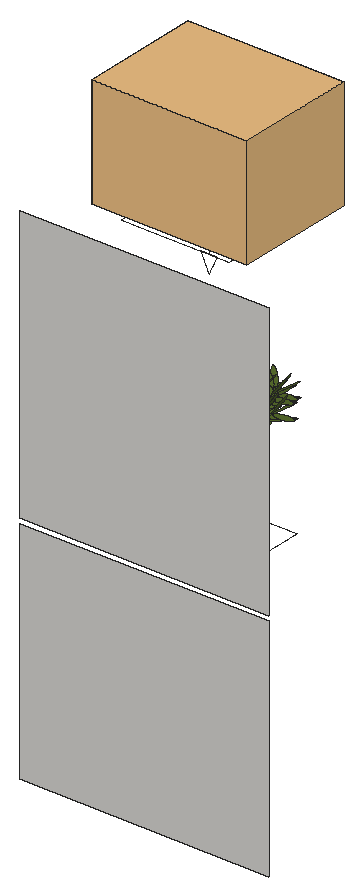
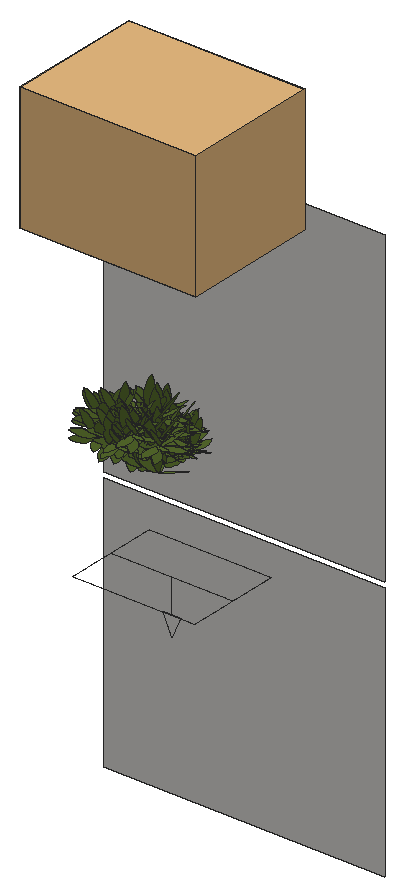
# SketchUp Ruby script. Lengths in inches.
U = 1.inch
M = Sketchup.active_model
def pt(a) = Geom::Point3d.new(a.map { |v| v * U })
def face(e, loops, mat)
  f = e.add_face(loops[0].map { |a| pt(a) })
  loops[1..].each { |l| e.add_face(l.map { |a| pt(a) }).erase! }
  f.material = f.back_material = mat if mat
  f
end
# faces: each face lists its corners as indices into pts; further lists are holes
def faces(e, pts, list, mat = nil) = list.each { |f| face(e, (f[0].is_a?(Array) ? f : [f]).map { |l| l.map { |i| pts[i] } }, mat) }
# xy, xz, yz: faces in a plane at the given z, y or x. An outline is a flat list of corners, or four numbers for a rectangle; further outlines are holes
def ring(l) = l.size == 4 ? [[l[0], l[1]], [l[2], l[1]], [l[2], l[3]], [l[0], l[3]]] : l.each_slice(2).to_a
def flat(e, list, mat, &to3) = list.each { |f| face(e, (f[0].is_a?(Array) ? f : [f]).map { |l| ring(l).map { |u, v| to3.(u, v) } }, mat) }
def xy(e, z, list, mat = nil) = flat(e, list, mat) { |x, y| [x, y, z] }
def xz(e, y, list, mat = nil) = flat(e, list, mat) { |x, z| [x, y, z] }
def yz(e, x, list, mat = nil) = flat(e, list, mat) { |y, z| [x, y, z] }
def lines(e, pts, list) = list.each { |a, b| e.add_line(pt(pts[a]), pt(pts[b])) }
# prism: a flat outline (further loops are holes) pulled along v
def prism(e, loops, v, mat = nil)
  f = face(e, loops, mat); d = Geom::Vector3d.new(v.map { |x| x * U })
  f.pushpull(f.normal.samedirection?(d) ? d.length : -d.length)
end
def box(e, o, s, mat = nil) = prism(e, [[o, [o[0] + s[0], o[1], o[2]], [o[0] + s[0], o[1] + s[1], o[2]], [o[0], o[1] + s[1], o[2]]]], [0, 0, s[2]], mat)
def at(x, y, z, deg = 0) = Geom::Transformation.translation(pt([x, y, z])) * Geom::Transformation.rotation(ORIGIN, Z_AXIS, deg.degrees)
def axes(o, x, y, z) = Geom::Transformation.new([*x, 0, *y, 0, *z, 0, *pt(o).to_a, 1])
def part(name) = M.definitions.add(name)
# library, detail: a bought-in or finely detailed component or shape, given as its bounding box
def library(name, o, s) = part(name).tap { |d| box(d.entities, o, s) }
def detail(e, o, s) = box(e.add_group.entities, o, s)
def put(e, d, t, mat = nil) = e.add_instance(d, t).tap { |i| i.material = mat if mat }
def group(e, t, mat = nil) = e.add_group.tap { |g| g.transformation = t; g.material = mat if mat }.entities
root = M.entities
M.materials.add("[0008_LavenderBlush]").color = [212, 210, 207]
M.materials.add("[Asphalt_New]").color = [85, 106, 44]
M.materials.add("white").color = [255, 255, 255]
c1 = library("Hanging planter",[0,-5.51,0],[18.9,24.41,17.52])
c2 = part("Component\#59")
xy(c2.entities,0,[[5.79,0,4.75,0.06,3.73,0.22,2.73,0.5,1.77,0.88,0.86,1.37,0,1.95,0.83,2.59,1.74,3.13,2.7,3.56,3.7,3.87,4.74,4.05,5.79,4.12,6.84,4.05,7.87,3.87,8.88,3.56,9.84,3.13,10.74,2.59,11.57,1.95,10.72,1.37,9.8,0.88,8.84,0.5,7.84,0.22,6.82,0.06]],"[Asphalt_New]")
c3 = part("Leaf cluster")
put(c3.entities,c2,axes([10.37,9.23,1.73],[-0.67725,-0.67301,0.29729],[0.61625,-0.73963,-0.27052],[0.40195,0,0.91566]),"[Asphalt_New]")
put(c3.entities,c2,at(0,5.84,1.2),"[Asphalt_New]")
put(c3.entities,c2,axes([11.625,9.72,1.52],[-0.61694,-0.11161,0.77906],[-0.02647,-0.98639,-0.16227],[0.78657,-0.12073,0.60559]),"[Asphalt_New]")
put(c3.entities,c2,axes([13.35,8.05,1.98],[-0.1211,0.99122,-0.05316],[-0.90762,-0.13226,-0.39842],[-0.40195,0,0.91566]),"[Asphalt_New]")
c4 = part("Group141\#1")
p = [[0,0,0],[0,0,-2.45],[-0.68,0,-2.45],[4.45,-3.49,0],[-4.45,-3.49,0],[4.45,3.49,0],
  [4.45,0,0],[-4.45,3.49,0],[0.68,0,-2.45],[-4.45,0,0],[0,0,-3.97]]
lines(c4.entities,p,[[0,1],[1,2],[3,4],[5,6],[7,5],[1,8],[9,0],[0,6],[8,10],[4,9],[6,3],[2,10],
  [9,7]])
c5 = part("Rectangle Light")
put(c5.entities,c4,at(0,0,0))
c6 = part("Groupe\#6")
put(c6.entities,c3,axes([6.2,8.72,2.56],[0.20072,0.20931,0],[-0.20931,0.20072,0],[0,0,0.3393]))
put(c6.entities,c3,axes([3.21,14.77,2.82],[0.12393,-0.26218,0],[0.26218,0.12393,0],[0,0,0.3393]))
put(c6.entities,c2,axes([6.98,12.58,2.74],[0.18147,-0.01125,0.26433],[0.07569,0.27597,-0.05506],[-0.21317,0.08841,0.20548]),"[Asphalt_New]")
put(c6.entities,c3,axes([9.62,7.71,2.12],[0.13301,0.2577,0],[-0.2577,0.13301,0],[0,0,0.3393]))
put(c6.entities,c3,axes([5.04,12.65,2.375],[0.19329,-0.21619,0],[0.21619,0.19329,0],[0,0,0.3393]))
put(c6.entities,c3,axes([8.55,8.27,2.12],[0.13301,0.2577,0],[-0.2577,0.13301,0],[0,0,0.3393]))
put(c6.entities,c3,axes([3.97,13.21,2.375],[0.19329,-0.21619,0],[0.21619,0.19329,0],[0,0,0.3393]))
put(c6.entities,c3,axes([13.2,6.93,2.95],[-0.24238,0.15922,0],[-0.15922,-0.24238,0],[0,0,0.3393]))
put(c6.entities,c3,axes([7.8,2.89,3.21],[0.23521,0.16964,0],[-0.16964,0.23521,0],[0,0,0.3393]))
put(c6.entities,c2,axes([9.26,7,3.13],[-0.02201,0.18048,0.26433],[-0.28514,0.02413,-0.05506],[-0.04808,-0.22571,0.20548]),"[Asphalt_New]")
put(c6.entities,c3,axes([10.92,8.49,3.88],[-0.24238,0.15922,0],[-0.15922,-0.24238,0],[0,0,0.3393]))
put(c6.entities,c3,axes([5.52,4.45,4.14],[0.23521,0.16964,0],[-0.16964,0.23521,0],[0,0,0.3393]))
put(c6.entities,c2,axes([6.97,8.56,4.0625],[-0.02201,0.18048,0.26433],[-0.28514,0.02413,-0.05506],[-0.04808,-0.22571,0.20548]),"[Asphalt_New]")
put(c6.entities,c3,axes([9.9,10.06,2.52],[-0.24238,0.15922,0],[-0.15922,-0.24238,0],[0,0,0.3393]))
put(c6.entities,c3,axes([4.51,6.02,2.78],[0.23521,0.16964,0],[-0.16964,0.23521,0],[0,0,0.3393]))
put(c6.entities,c2,axes([5.96,10.125,2.71],[-0.02201,0.18048,0.26433],[-0.28514,0.02413,-0.05506],[-0.04808,-0.22571,0.20548]),"[Asphalt_New]")
put(c6.entities,c3,axes([13.6,14.86,2.41],[-0.24779,-0.15066,0],[0.15066,-0.24779,0],[0,0,0.3393]))
put(c6.entities,c3,axes([8.65,12.2,2.15],[0.22914,-0.17774,0],[0.17774,0.22914,0],[0,0,0.3393]))
put(c6.entities,c3,axes([14.35,15.81,2.41],[-0.24779,-0.15066,0],[0.15066,-0.24779,0],[0,0,0.3393]))
put(c6.entities,c3,axes([7.9,11.25,2.15],[0.22914,-0.17774,0],[0.17774,0.22914,0],[0,0,0.3393]))
put(c6.entities,c3,axes([-0.46,12.1,3.24],[0.12393,-0.26218,0],[0.26218,0.12393,0],[0,0,0.3393]))
put(c6.entities,c2,axes([3.31,9.91,3.17],[0.18147,-0.01125,0.26433],[0.07569,0.27597,-0.05506],[-0.21317,0.08841,0.20548]),"[Asphalt_New]")
put(c6.entities,c3,axes([4.47,8.01,3.91],[0.20072,0.20931,0],[-0.20931,0.20072,0],[0,0,0.3393]))
put(c6.entities,c3,axes([1.49,14.06,4.17],[0.12393,-0.26218,0],[0.26218,0.12393,0],[0,0,0.3393]))
put(c6.entities,c2,axes([5.26,11.88,4.1],[0.18147,-0.01125,0.26433],[0.07569,0.27597,-0.05506],[-0.21317,0.08841,0.20548]),"[Asphalt_New]")
put(c6.entities,c3,axes([6.85,4.1,2.54],[0.13301,0.2577,0],[-0.2577,0.13301,0],[0,0,0.3393]))
put(c6.entities,c3,axes([2.27,9.05,2.8],[0.19329,-0.21619,0],[0.21619,0.19329,0],[0,0,0.3393]))
put(c6.entities,c2,axes([6.51,8.03,2.73],[0.17719,0.04076,0.26433],[-0.00581,0.2861,-0.05506],[-0.2295,0.02423,0.20548]),"[Asphalt_New]")
put(c6.entities,c3,axes([4.86,14.63,2.58],[0.22914,-0.17774,0],[0.17774,0.22914,0],[0,0,0.3393]))
put(c6.entities,c3,axes([10.5625,18.23,2.83],[-0.24779,-0.15066,0],[0.15066,-0.24779,0],[0,0,0.3393]))
put(c6.entities,c2,axes([8.79,14.25,2.76],[0.00779,-0.18165,0.26433],[0.28237,-0.04643,-0.05506],[0.06564,0.22124,0.20548]),"[Asphalt_New]")
put(c6.entities,c3,axes([7.02,12.9,3.51],[0.22914,-0.17774,0],[0.17774,0.22914,0],[0,0,0.3393]))
put(c6.entities,c3,axes([12.72,16.5,3.76],[-0.24779,-0.15066,0],[0.15066,-0.24779,0],[0,0,0.3393]))
put(c6.entities,c2,axes([10.94,12.52,3.6875],[0.00779,-0.18165,0.26433],[0.28237,-0.04643,-0.05506],[0.06564,0.22124,0.20548]),"[Asphalt_New]")
put(c6.entities,c3,axes([5.98,10.15,2.19],[0.23521,0.16964,0],[-0.16964,0.23521,0],[0,0,0.3393]))
put(c6.entities,c3,axes([9.23,9.05,2.52],[-0.24238,0.15922,0],[-0.15922,-0.24238,0],[0,0,0.3393]))
put(c6.entities,c3,axes([3.84,5.01,2.78],[0.23521,0.16964,0],[-0.16964,0.23521,0],[0,0,0.3393]))
put(c6.entities,c2,axes([5.29,9.12,2.71],[-0.02201,0.18048,0.26433],[-0.28514,0.02413,-0.05506],[-0.04808,-0.22571,0.20548]),"[Asphalt_New]")
put(c6.entities,c3,axes([4.09,12.81,2.58],[0.23461,-0.17046,0],[0.17046,0.23461,0],[0,0,0.3393]))
put(c6.entities,c3,axes([9.68,16.59,2.83],[-0.24294,-0.15837,0],[0.15837,-0.24294,0],[0,0,0.3393]))
put(c6.entities,c2,axes([8.03,12.56,2.76],[0.01349,-0.18132,0.26433],[0.28368,-0.03753,-0.05506],[0.05866,0.22319,0.20548]),"[Asphalt_New]")
put(c6.entities,c3,axes([6.3,11.15,3.51],[0.23461,-0.17046,0],[0.17046,0.23461,0],[0,0,0.3393]))
put(c6.entities,c3,axes([11.89,14.93,3.76],[-0.24294,-0.15837,0],[0.15837,-0.24294,0],[0,0,0.3393]))
put(c6.entities,c2,axes([10.24,10.89,3.6875],[0.01349,-0.18132,0.26433],[0.28368,-0.03753,-0.05506],[0.05866,0.22319,0.20548]),"[Asphalt_New]")
put(c6.entities,c3,axes([11.75,13.77,2.17],[-0.145,-0.25115,0],[0.25115,-0.145,0],[0,0,0.3393]))
put(c6.entities,c3,axes([16.09,8.62,2.43],[-0.1829,0.22505,0],[-0.22505,-0.1829,0],[0,0,0.3393]))
put(c6.entities,c3,axes([10.33,11.4,3.1],[-0.145,-0.25115,0],[0.25115,-0.145,0],[0,0,0.3393]))
put(c6.entities,c3,axes([14.67,6.25,3.36],[-0.1829,0.22505,0],[-0.22505,-0.1829,0],[0,0,0.3393]))
put(c6.entities,c2,axes([10.48,7.46,3.28],[-0.17891,-0.03237,0.26433],[-0.00768,-0.28605,-0.05506],[0.2281,-0.03501,0.20548]),"[Asphalt_New]")
put(c6.entities,c3,axes([7.24,9.53,2.15],[0.23461,-0.17046,0],[0.17046,0.23461,0],[0,0,0.3393]))
put(c6.entities,c3,axes([12.82,13.3125,2.41],[-0.24294,-0.15837,0],[0.15837,-0.24294,0],[0,0,0.3393]))
put(c6.entities,c3,axes([7.96,10.51,2.15],[0.23461,-0.17046,0],[0.17046,0.23461,0],[0,0,0.3393]))
put(c6.entities,c3,axes([13.54,14.29,2.41],[-0.24294,-0.15837,0],[0.15837,-0.24294,0],[0,0,0.3393]))
put(c6.entities,c3,axes([10,6.52,1.96],[0.20072,0.20931,0],[-0.20931,0.20072,0],[0,0,0.3393]))
put(c6.entities,c3,axes([7.01,12.5625,2.22],[0.12393,-0.26218,0],[0.26218,0.12393,0],[0,0,0.3393]))
put(c6.entities,c3,axes([5.33,9.5625,2.56],[0.20072,0.20931,0],[-0.20931,0.20072,0],[0,0,0.3393]))
put(c6.entities,c3,axes([2.34,15.61,2.82],[0.12393,-0.26218,0],[0.26218,0.12393,0],[0,0,0.3393]))
put(c6.entities,c2,axes([6.12,13.43,2.74],[0.18147,-0.01125,0.26433],[0.07569,0.27597,-0.05506],[-0.21317,0.08841,0.20548]),"[Asphalt_New]")
put(c6.entities,c3,axes([13.16,5.15,2],[-0.1829,0.22505,0],[-0.22505,-0.1829,0],[0,0,0.3393]))
put(c6.entities,c3,axes([14.2,4.53,2],[-0.1829,0.22505,0],[-0.22505,-0.1829,0],[0,0,0.3393]))
put(c6.entities,c3,axes([8.17,6.54,3.47],[0.13301,0.2577,0],[-0.2577,0.13301,0],[0,0,0.3393]))
put(c6.entities,c3,axes([3.58,11.48,3.73],[0.19329,-0.21619,0],[0.21619,0.19329,0],[0,0,0.3393]))
put(c6.entities,c2,axes([7.82,10.46,3.66],[0.17719,0.04076,0.26433],[-0.00581,0.2861,-0.05506],[-0.2295,0.02423,0.20548]),"[Asphalt_New]")
put(c6.entities,c3,axes([2.52,6.05,2.98],[0.20072,0.20931,0],[-0.20931,0.20072,0],[0,0,0.3393]))
xz(root,9,[[127.1875,41,147.625,59.82],[127.1875,60.22,147.625,82.88]],"[0008_LavenderBlush]")
put(root,c1,axes([133.55,21.88,83.28],[0,-0.52438,0],[0.52438,0,0],[0,0,0.52438]),"white")
put(root,c2,axes([137.25,14.88,67.86],[0.01807,0.15078,-0.00946],[-0.13884,0.01339,-0.07089],[-0.05936,0.01458,0.16292]),"[Asphalt_New]")
put(root,c3,axes([138.78,17.14,67.59],[-0.10136,0.11337,0],[-0.11337,-0.10136,0],[0,0,0.17792]),"white")
put(root,c2,axes([136.21,15.24,68.18],[0.15184,-0.00221,-0.00946],[-0.00119,0.13948,-0.07089],[0.0083,0.06056,0.16292]),"[Asphalt_New]")
put(root,c2,axes([137.7,16.39,67.82],[-0.12443,-0.07482,0.0529],[0.06418,-0.13158,-0.04813],[0.05936,-0.01458,0.16292]),"[Asphalt_New]")
put(root,c2,axes([137.96,15.16,67.85],[-0.15155,-0.00971,-0.00946],[0.01213,-0.13895,-0.07089],[-0.00352,-0.06102,0.16292]),"[Asphalt_New]")
put(root,c2,axes([137.45,12.3,67.5],[0.00875,0.15182,0],[-0.15182,0.00875,0],[0,0,0.17792]),"[Asphalt_New]")
put(root,c2,axes([137.01,16.93,68.75],[-0.02064,-0.15066,0],[0.15066,-0.02064,0],[0,0,0.17792]),"[Asphalt_New]")
put(root,c3,axes([135.63,14.95,67.67],[0.1271,-0.08349,0],[0.08349,0.1271,0],[0,0,0.17792]),"white")
put(root,c2,axes([137.9,16.41,67.78],[-0.09516,0.0059,0.13861],[-0.03969,-0.14471,-0.02887],[0.11178,-0.04636,0.10775]),"[Asphalt_New]")
put(root,c2,axes([137.53,13.33,67.71],[0.00875,0.15182,0],[-0.15182,0.00875,0],[0,0,0.17792]),"[Asphalt_New]")
put(root,c3,axes([138.92,16.15,68],[-0.12303,0.08939,0],[-0.08939,-0.12303,0],[0,0,0.17792]),"white")
put(root,c3,axes([138.95,15.76,68],[-0.12016,0.09321,0],[-0.09321,-0.12016,0],[0,0,0.17792]),"white")
put(root,c2,axes([136.96,14.1,67.55],[0.01154,-0.09464,0.13861],[0.14952,-0.01265,-0.02887],[0.02521,0.11836,0.10775]),"[Asphalt_New]")
put(root,c2,axes([136.49,14.89,68.02],[0.1519,0.00716,0],[-0.00716,0.1519,0],[0,0,0.17792]),"[Asphalt_New]")
put(root,c3,axes([139.03,14.04,67.82],[-0.06499,0.13748,0],[-0.13748,-0.06499,0],[0,0,0.17792]),"white")
put(root,c2,axes([137.73,15.95,68.81],[-0.00707,0.09508,0.13861],[-0.14876,0.01968,-0.02887],[-0.03076,-0.11704,0.10775]),"[Asphalt_New]")
put(root,c2,axes([136.85,16.51,68.1],[0.09382,0.01697,0.13861],[0.00402,0.15,-0.02887],[-0.11961,0.01836,0.10775]),"[Asphalt_New]")
put(root,c2,axes([137.04,15.13,67.77],[0.01154,-0.09464,0.13861],[0.14952,-0.01265,-0.02887],[0.02521,0.11836,0.10775]),"[Asphalt_New]")
put(root,c5,at(137.45,15.57,59.82,180))
put(root,c5,at(137.45,15.57,82.88,180))
put(root,c2,axes([136.58,16.05,68.18],[0.15183,0.00256,-0.00946],[-0.00557,0.13937,-0.07089],[0.00639,0.06079,0.16292]),"[Asphalt_New]")
put(root,c2,axes([137.63,15.91,68.08],[0.01807,0.15078,-0.00946],[-0.13884,0.01339,-0.07089],[-0.05936,0.01458,0.16292]),"[Asphalt_New]")
put(root,c2,axes([136.61,15.74,68.18],[0.15184,-0.00221,-0.00946],[-0.00119,0.13948,-0.07089],[0.0083,0.06056,0.16292]),"[Asphalt_New]")
put(root,c2,axes([137.33,17.77,68.75],[-0.0159,-0.15124,0],[0.15124,-0.0159,0],[0,0,0.17792]),"[Asphalt_New]")
put(root,c2,axes([138.22,17.54,67.82],[-0.12443,-0.07482,0.0529],[0.06418,-0.13158,-0.04813],[0.05936,-0.01458,0.16292]),"[Asphalt_New]")
put(root,c2,axes([138.4,15.11,67.58],[-0.08742,0.11593,0.0529],[-0.12415,-0.07758,-0.04813],[-0.0083,-0.06056,0.16292]),"[Asphalt_New]")
put(root,c3,axes([137.52,12.83,67.58],[0.12994,0.079,0],[-0.079,0.12994,0],[0,0,0.17792]),"white")
put(root,c3,axes([139.3,16.67,68],[-0.12303,0.08939,0],[-0.08939,-0.12303,0],[0,0,0.17792]),"white")
put(root,c2,axes([138.44,14.39,68.36],[-0.08742,0.11593,0.0529],[-0.12415,-0.07758,-0.04813],[-0.0083,-0.06056,0.16292]),"[Asphalt_New]")
put(root,c2,axes([138.04,15.48,68.11],[-0.09806,-0.10708,0.0529],[0.09891,-0.10794,-0.04813],[0.06106,0.00288,0.16292]),"[Asphalt_New]")
put(root,c2,axes([137.3,16.9,67.41],[0.01842,-0.15074,-0.00946],[0.13802,0.02011,-0.07089],[0.06112,0,0.16292]),"[Asphalt_New]")
put(root,c3,axes([137.72,16.25,67.59],[-0.12334,-0.08896,0],[0.08896,-0.12334,0],[0,0,0.17792]),"white")
put(root,c2,axes([138.23,15.5625,68.08],[-0.09292,-0.02137,0.13861],[0.00305,-0.15002,-0.02887],[0.12035,-0.0127,0.10775]),"[Asphalt_New]")
put(root,c2,axes([137.98,12,67.71],[0.00875,0.15182,0],[-0.15182,0.00875,0],[0,0,0.17792]),"[Asphalt_New]")
put(root,c3,axes([137.56,12.1,68.36],[0.12994,0.079,0],[-0.079,0.12994,0],[0,0,0.17792]),"white")
put(root,c2,axes([138.62,17.1,68.05],[-0.15207,0,0],[0,-0.15207,0],[0,0,0.17792]),"[Asphalt_New]")
put(root,c3,axes([137.46,17.21,67.6875],[-0.10525,-0.10976,0],[0.10976,-0.10525,0],[0,0,0.17792]),"white")
put(root,c3,axes([139.42,15.08,68.04],[-0.06499,0.13748,0],[-0.13748,-0.06499,0],[0,0,0.17792]),"white")
put(root,c3,axes([139.41,14.9,68.71],[-0.12016,0.09321,0],[-0.09321,-0.12016,0],[0,0,0.17792]),"white")
put(root,c3,axes([137.81,17.29,67.81],[-0.12334,-0.08896,0],[0.08896,-0.12334,0],[0,0,0.17792]),"white")
put(root,c2,axes([137.02,13.91,67.59],[0.09625,-0.10871,0.0529],[0.11768,0.08708,-0.04813],[0.00352,0.06102,0.16292]),"[Asphalt_New]")
put(root,c2,axes([136.96,16.56,68.18],[0.15183,0.00256,-0.00946],[-0.00557,0.13937,-0.07089],[0.00639,0.06079,0.16292]),"[Asphalt_New]")
put(root,c2,axes([137.49,13.8,67.77],[0.01154,-0.09464,0.13861],[0.14952,-0.01265,-0.02887],[0.02521,0.11836,0.10775]),"[Asphalt_New]")
put(root,c2,axes([137.1,14.9375,67.8],[0.09625,-0.10871,0.0529],[0.11768,0.08708,-0.04813],[0.00352,0.06102,0.16292]),"[Asphalt_New]")
put(root,c2,axes([138.09,16.1,67.86],[0.01807,0.15078,-0.00946],[-0.13884,0.01339,-0.07089],[-0.05936,0.01458,0.16292]),"[Asphalt_New]")
put(root,c2,axes([137.05,14.6,68.02],[0.1519,0.00716,0],[-0.00716,0.1519,0],[0,0,0.17792]),"[Asphalt_New]")
put(root,c2,axes([138.18,13.11,67.71],[0.00875,0.15182,0],[-0.15182,0.00875,0],[0,0,0.17792]),"[Asphalt_New]")
put(root,c2,axes([137.07,14.875,68.89],[0.15184,-0.00221,-0.00946],[-0.00119,0.13948,-0.07089],[0.0083,0.06056,0.16292]),"[Asphalt_New]")
put(root,c2,axes([138.77,16,67.58],[-0.09102,0.11312,0.0529],[-0.12166,-0.08144,-0.04813],[-0.00639,-0.06079,0.16292]),"[Asphalt_New]")
put(root,c2,axes([138.83,15.28,68.36],[-0.09102,0.11312,0.0529],[-0.12166,-0.08144,-0.04813],[-0.00639,-0.06079,0.16292]),"[Asphalt_New]")
put(root,c3,axes([137.96,13.69,67.58],[0.12739,0.08305,0],[-0.08305,0.12739,0],[0,0,0.17792]),"white")
put(root,c2,axes([137.69,14.91,67.77],[0.01154,-0.09464,0.13861],[0.14952,-0.01265,-0.02887],[0.02521,0.11836,0.10775]),"[Asphalt_New]")
put(root,c2,axes([138.5,15.32,68.16],[-0.0255,0.1497,-0.00946],[-0.13692,-0.02659,-0.07089],[-0.06106,-0.00288,0.16292]),"[Asphalt_New]")
put(root,c2,axes([138.95,13.46,67.85],[-0.15155,-0.00971,-0.00946],[0.01213,-0.13895,-0.07089],[-0.00352,-0.06102,0.16292]),"[Asphalt_New]")
put(root,c2,axes([137.24,16.61,67.47],[0.1519,0.00716,0],[-0.00716,0.1519,0],[0,0,0.17792]),"[Asphalt_New]")
put(root,c2,axes([137.5625,16.64,67.33],[0.09382,0.01697,0.13861],[0.00402,0.15,-0.02887],[-0.11961,0.01836,0.10775]),"[Asphalt_New]")
put(root,c2,axes([138.45,14.91,67.54],[-0.00408,0.09525,0.13861],[-0.14807,0.02435,-0.02887],[-0.03442,-0.11602,0.10775]),"[Asphalt_New]")
put(root,c2,axes([137.26,15.5,68.73],[0.1519,0.00716,0],[-0.00716,0.1519,0],[0,0,0.17792]),"[Asphalt_New]")
put(root,c3,axes([138.02,12.96,68.36],[0.12739,0.08305,0],[-0.08305,0.12739,0],[0,0,0.17792]),"white")
put(root,c3,axes([137.85,18.25,67.9],[-0.10525,-0.10976,0],[0.10976,-0.10525,0],[0,0,0.17792]),"white")
put(root,c2,axes([138.49,14.19,68.32],[-0.00408,0.09525,0.13861],[-0.14807,0.02435,-0.02887],[-0.03442,-0.11602,0.10775]),"[Asphalt_New]")
put(root,c3,axes([139.79,15.82,68.71],[-0.12303,0.08939,0],[-0.08939,-0.12303,0],[0,0,0.17792]),"white")
put(root,c3,axes([136.61,13.25,67.67],[0.1271,-0.08349,0],[0.08349,0.1271,0],[0,0,0.17792]),"white")
put(root,c3,axes([139.875,15.27,67.82],[-0.06499,0.13748,0],[-0.13748,-0.06499,0],[0,0,0.17792]),"white")
put(root,c3,axes([138.25,15.96,67.81],[-0.12334,-0.08896,0],[0.08896,-0.12334,0],[0,0,0.17792]),"white")
put(root,c2,axes([138.61,15.1875,68.11],[-0.09806,-0.10708,0.0529],[0.09891,-0.10794,-0.04813],[0.06106,0.00288,0.16292]),"[Asphalt_New]")
put(root,c2,axes([138.79,15.27,68.08],[-0.09292,-0.02137,0.13861],[0.00305,-0.15002,-0.02887],[0.12035,-0.0127,0.10775]),"[Asphalt_New]")
put(root,c2,axes([138.1,16.75,67.49],[-0.02064,-0.15066,0],[0.15066,-0.02064,0],[0,0,0.17792]),"[Asphalt_New]")
put(root,c2,axes([137.45,15.72,68.89],[0.15183,0.00256,-0.00946],[-0.00557,0.13937,-0.07089],[0.00639,0.06079,0.16292]),"[Asphalt_New]")
put(root,c2,axes([138.14,16.02,68.26],[-0.02064,-0.15066,0],[0.15066,-0.02064,0],[0,0,0.17792]),"[Asphalt_New]")
put(root,c2,axes([139.19,14.85,67.85],[-0.15155,-0.00971,-0.00946],[0.01213,-0.13895,-0.07089],[-0.00352,-0.06102,0.16292]),"[Asphalt_New]")
put(root,c2,axes([137.55,13.61,67.8],[0.09625,-0.10871,0.0529],[0.11768,0.08708,-0.04813],[0.00352,0.06102,0.16292]),"[Asphalt_New]")
put(root,c2,axes([138.79,17.2,67.5625],[-0.09806,-0.10708,0.0529],[0.09891,-0.10794,-0.04813],[0.06106,0.00288,0.16292]),"[Asphalt_New]")
put(root,c3,axes([138.46,17.0625,67.81],[-0.12334,-0.08896,0],[0.08896,-0.12334,0],[0,0,0.17792]),"white")
put(root,c2,axes([138.81,16.09,68.83],[-0.09806,-0.10708,0.0529],[0.09891,-0.10794,-0.04813],[0.06106,0.00288,0.16292]),"[Asphalt_New]")
put(root,c2,axes([138.98,17.28,67.53],[-0.09292,-0.02137,0.13861],[0.00305,-0.15002,-0.02887],[0.12035,-0.0127,0.10775]),"[Asphalt_New]")
put(root,c2,axes([139.33,17.23,67.27],[-0.15207,0,0],[0,-0.15207,0],[0,0,0.17792]),"[Asphalt_New]")
put(root,c3,axes([136.85,14.64,67.67],[0.1271,-0.08349,0],[0.08349,0.1271,0],[0,0,0.17792]),"white")
put(root,c2,axes([138.99,16.18,68.79],[-0.09292,-0.02137,0.13861],[0.00305,-0.15002,-0.02887],[0.12035,-0.0127,0.10775]),"[Asphalt_New]")
put(root,c2,axes([138.82,15.8,67.54],[-0.00707,0.09508,0.13861],[-0.14876,0.01968,-0.02887],[-0.03076,-0.11704,0.10775]),"[Asphalt_New]")
put(root,c3,axes([140.13,17.43,67.47],[-0.12016,0.09321,0],[-0.09321,-0.12016,0],[0,0,0.17792]),"white")
put(root,c3,axes([138.34,15.14,67.61],[0.12994,0.079,0],[-0.079,0.12994,0],[0,0,0.17792]),"white")
put(root,c2,axes([137.58,14.91,68.25],[0.14768,-0.03627,0],[0.03627,0.14768,0],[0,0,0.17792]),"[Asphalt_New]")
put(root,c2,axes([138.89,15.08,68.32],[-0.00707,0.09508,0.13861],[-0.14876,0.01968,-0.02887],[-0.03076,-0.11704,0.10775]),"[Asphalt_New]")
put(root,c2,axes([137.76,14.71,67.8],[0.09625,-0.10871,0.0529],[0.11768,0.08708,-0.04813],[0.00352,0.06102,0.16292]),"[Asphalt_New]")
put(root,c2,axes([138.82,15.48,67.68],[0.00875,0.15182,0],[-0.15182,0.00875,0],[0,0,0.17792]),"[Asphalt_New]")
put(root,c3,axes([138.31,18.4375,67.6875],[-0.10525,-0.10976,0],[0.10976,-0.10525,0],[0,0,0.17792]),"white")
put(root,c2,axes([139.46,14.43,68.0625],[-0.15155,-0.00971,-0.00946],[0.01213,-0.13895,-0.07089],[-0.00352,-0.06102,0.16292]),"[Asphalt_New]")
put(root,c2,axes([139.07,15.03,68.16],[-0.0255,0.1497,-0.00946],[-0.13692,-0.02659,-0.07089],[-0.06106,-0.00288,0.16292]),"[Asphalt_New]")
put(root,c2,axes([138.42,17.62,67.49],[-0.0159,-0.15124,0],[0.15124,-0.0159,0],[0,0,0.17792]),"[Asphalt_New]")
put(root,c2,axes([139.23,15.04,68.34],[-0.12443,-0.07482,0.0529],[0.06418,-0.13158,-0.04813],[0.05936,-0.01458,0.16292]),"[Asphalt_New]")
put(root,c6,axes([132.83,13.8,67.9],[0.48162,-0.20742,0],[0.20742,0.48162,0],[0,0,0.52438]),"white")
put(root,c2,axes([138.48,16.9,68.26],[-0.0159,-0.15124,0],[0.15124,-0.0159,0],[0,0,0.17792]),"[Asphalt_New]")
put(root,c2,axes([138.34,17.28,67.74],[0.01154,-0.09464,0.13861],[0.14952,-0.01265,-0.02887],[0.02521,0.11836,0.10775]),"[Asphalt_New]")
put(root,c3,axes([137.13,14.22,67.88],[0.1271,-0.08349,0],[0.08349,0.1271,0],[0,0,0.17792]),"white")
put(root,c3,axes([140.4,16.42,67.82],[-0.06499,0.13748,0],[-0.13748,-0.06499,0],[0,0,0.17792]),"white")
put(root,c3,axes([140.45,15.03,68.12],[-0.10136,0.11337,0],[-0.11337,-0.10136,0],[0,0,0.17792]),"white")
put(root,c3,axes([138.05,17.62,67.98],[-0.06975,-0.13513,0],[0.13513,-0.06975,0],[0,0,0.17792]),"white")
put(root,c2,axes([139.43,15.0625,68.31],[-0.09516,0.0059,0.13861],[-0.03969,-0.14471,-0.02887],[0.11178,-0.04636,0.10775]),"[Asphalt_New]")
put(root,c2,axes([139.27,15.94,68.87],[-0.0255,0.1497,-0.00946],[-0.13692,-0.02659,-0.07089],[-0.06106,-0.00288,0.16292]),"[Asphalt_New]")
